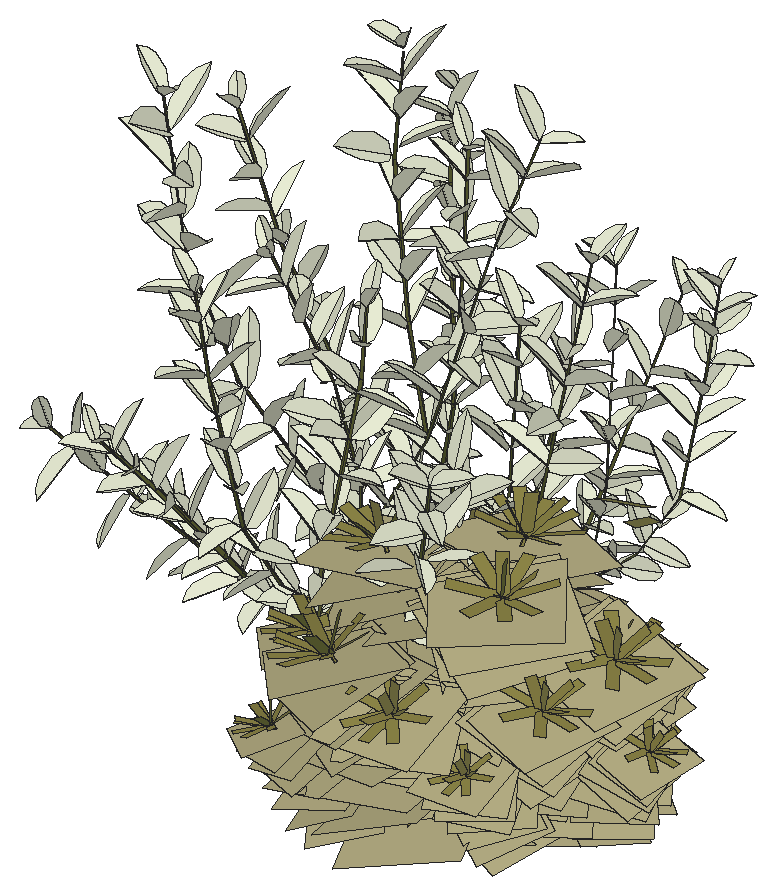
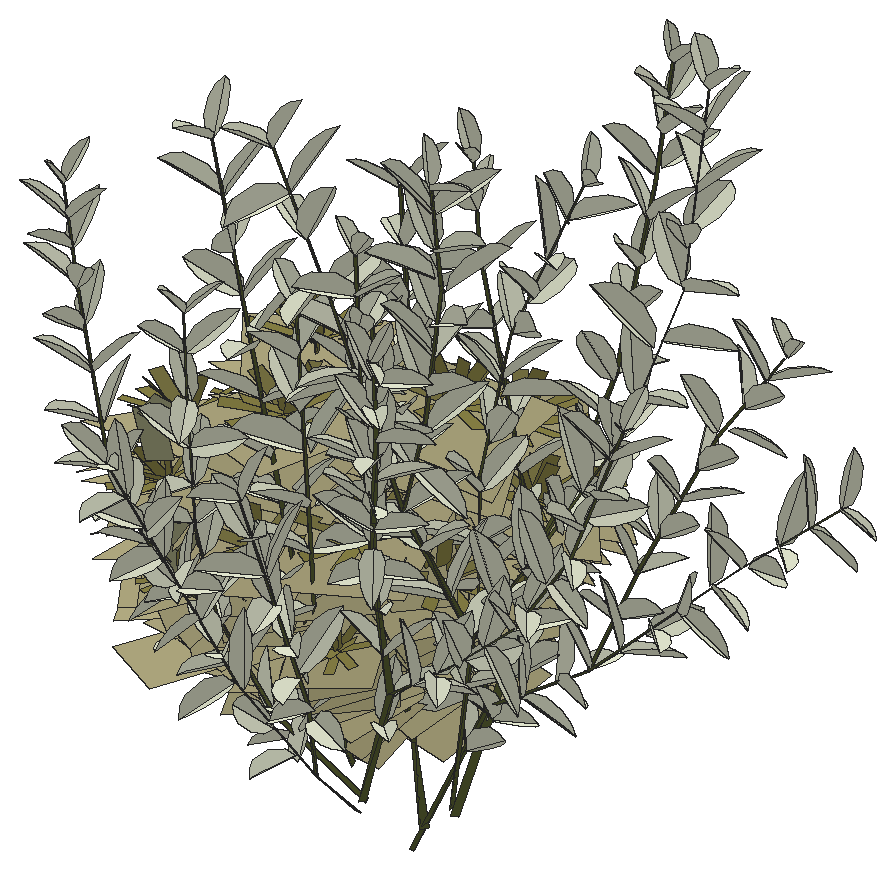
# SketchUp Ruby script. Lengths in inches.
U = 1.inch
M = Sketchup.active_model
def pt(a) = Geom::Point3d.new(a.map { |v| v * U })
def face(e, loops, mat)
  f = e.add_face(loops[0].map { |a| pt(a) })
  loops[1..].each { |l| e.add_face(l.map { |a| pt(a) }).erase! }
  f.material = f.back_material = mat if mat
  f
end
# faces: each face lists its corners as indices into pts; further lists are holes
def faces(e, pts, list, mat = nil) = list.each { |f| face(e, (f[0].is_a?(Array) ? f : [f]).map { |l| l.map { |i| pts[i] } }, mat) }
# xy, xz, yz: faces in a plane at the given z, y or x. An outline is a flat list of corners, or four numbers for a rectangle; further outlines are holes
def ring(l) = l.size == 4 ? [[l[0], l[1]], [l[2], l[1]], [l[2], l[3]], [l[0], l[3]]] : l.each_slice(2).to_a
def flat(e, list, mat, &to3) = list.each { |f| face(e, (f[0].is_a?(Array) ? f : [f]).map { |l| ring(l).map { |u, v| to3.(u, v) } }, mat) }
def xy(e, z, list, mat = nil) = flat(e, list, mat) { |x, y| [x, y, z] }
def xz(e, y, list, mat = nil) = flat(e, list, mat) { |x, z| [x, y, z] }
def yz(e, x, list, mat = nil) = flat(e, list, mat) { |y, z| [x, y, z] }
def lines(e, pts, list) = list.each { |a, b| e.add_line(pt(pts[a]), pt(pts[b])) }
# prism: a flat outline (further loops are holes) pulled along v
def prism(e, loops, v, mat = nil)
  f = face(e, loops, mat); d = Geom::Vector3d.new(v.map { |x| x * U })
  f.pushpull(f.normal.samedirection?(d) ? d.length : -d.length)
end
def box(e, o, s, mat = nil) = prism(e, [[o, [o[0] + s[0], o[1], o[2]], [o[0] + s[0], o[1] + s[1], o[2]], [o[0], o[1] + s[1], o[2]]]], [0, 0, s[2]], mat)
def at(x, y, z, deg = 0) = Geom::Transformation.translation(pt([x, y, z])) * Geom::Transformation.rotation(ORIGIN, Z_AXIS, deg.degrees)
def axes(o, x, y, z) = Geom::Transformation.new([*x, 0, *y, 0, *z, 0, *pt(o).to_a, 1])
def part(name) = M.definitions.add(name)
# library, detail: a bought-in or finely detailed component or shape, given as its bounding box
def library(name, o, s) = part(name).tap { |d| box(d.entities, o, s) }
def detail(e, o, s) = box(e.add_group.entities, o, s)
def put(e, d, t, mat = nil) = e.add_instance(d, t).tap { |i| i.material = mat if mat }
def group(e, t, mat = nil) = e.add_group.tap { |g| g.transformation = t; g.material = mat if mat }.entities
root = M.entities
M.materials.add("0ad16as01f6asdLeafVar1sfd015as60f1as6").color = [231, 235, 211]
M.materials.add("Colorsadfasdfa0sd1f06w3").color = [153, 130, 61]
M.materials.add("Euphorbia asdfasd0f150160s159w").color = [180, 173, 131]
M.materials.add("Euphorbiaasdfa0sdf1a56sd016wow Leaf SU").color = [141, 134, 72]
M.materials.add("asdfasdf0165f6asdLeafVar1sfd015as60f1as6").color = [231, 235, 211]
M.materials.add("dw_stemssadfasdfa0sdf1s01d6w1").color = [90, 97, 50]
M.materials.add("viburnumbladsadfasdfad0w122").color = [125, 129, 119]
c1 = part("vdw_leaf\#1")
p = [[0,0,0],[-2.77,1.61,2.32],[-4.3125,6.1,4.5],[-3.97,13.49,6.09],[-2.47,18.57,6.3],[-0.2,22.73,5.75],
  [2.54,19.66,6.85],[4.3,15.93,7.09],[5.03,7.6,5.43],[3.32,1.76,2.74]]
faces(c1.entities,p,[[0,1,2,3,4,5],[0,5,6,7,8,9]],"0ad16as01f6asdLeafVar1sfd015as60f1as6")
c2 = part("dw_branch_3\#2")
p = [[-10.06,-1.6,62.9],[-0.2,1.54,-0.01],[-10.43,1.54,62.72],[0.18,-1.6,0.17],[-23.75,-21.66,88.91],[-25.7,-20.3,89.55],
  [13.4,11.62,104.56],[13.33,13.52,104.47],[-49.25,-41.87,130.3125],[-50.33,-40.21,130.71],[-4.97,21.13,143.98],[35.61,27.99,178.64],
  [-5.09,23.64,143.96],[35.32,29.14,178.46],[-67.7,-55.38,181.06],[-68.34,-54.45,181.62],[-22.8125,33.9,200.59],[-22.94,35.79,200.41],
  [56.61,36.78,229.75],[56.29,38.09,229.57],[-70.63,-67.46,248.85],[-70.72,-66.33,249.5],[-25.05,43.32,240.75],[-24.98,44.26,240.57]]
faces(c2.entities,p,[[0,1,2],[0,3,1],[4,2,5],[4,0,2],[6,0,2],[6,2,7],[8,4,5],[8,5,9],
  [10,6,7],[11,6,7],[10,7,12],[11,7,13],[14,8,9],[14,9,15],[16,10,12],[16,12,17],
  [18,11,13],[18,13,19],[20,14,15],[20,15,21],[22,16,17],[22,17,23]],"dw_stemssadfasdfa0sdf1s01d6w1")
c3 = part("dw_branch3\#2")
put(c3.entities,c1,axes([-70.33,-63.58,233.32],[-1.00752,0.412,0.78596],[-0.24851,-1.22189,0.32195],[0.83141,0.09817,1.01433]))
put(c3.entities,c1,axes([-66.93,-54.91,182.82],[-0.84976,-0.98359,0.33619],[0.99572,-0.74889,0.32577],[-0.05223,0.46521,1.22907]))
put(c3.entities,c1,axes([-46.12,-39.49,126.35],[1.23843,0.5364,0.23552],[-0.56438,0.94474,0.81599],[0.15707,-0.83465,1.07498]))
put(c3.entities,c1,axes([13.0625,13.13,104.77],[-1.01271,0.69982,-0.26884],[-0.74268,-0.99813,0.19939],[-0.10222,0.31872,1.21473]))
put(c3.entities,c1,axes([-18.87,30.42,186.42],[0.36309,1.06515,-0.56675],[-1.14134,0.49515,0.19939],[0.39128,0.45593,1.10754]))
put(c3.entities,c1,axes([-3.2,4.15,75.77],[-1.04153,0.55414,0.44243],[-0.23365,-1.01045,0.71554],[0.6695,0.50943,0.93801]))
put(c3.entities,c1,axes([23.2,19.41,136.3],[-0.65687,-1.11295,-0.05714],[1.05857,-0.61429,-0.20411],[0.15163,-0.1536,1.24868]))
put(c3.entities,c1,axes([-25.57,35.48,201.32],[-0.64726,0.62827,0.87973],[-0.71635,-1.0172,0.19939],[0.80962,-0.39773,0.87973]))
put(c3.entities,c1,axes([-36.37,-32.14,110.35],[-0.80747,1.09962,0.12544],[-0.83333,-0.50188,-0.96467],[-0.72833,-0.64487,0.96467]))
put(c3.entities,c1,axes([-9.89,26.72,156.79],[0.45529,1.02969,0.56572],[-1.16919,0.33753,0.32662],[0.11537,-0.64297,1.07744]))
put(c3.entities,c1,axes([-26.57,46.1,241.0625],[0.00015,0.80921,0.22536],[-0.83985,0.00446,-0.01542],[-0.01605,-0.22532,0.80906]))
put(c3.entities,c1,axes([-9.2,-2.58,61.06],[-1.10001,-0.40312,0.39014],[0.40883,-1.1116,0.00411],[0.35732,0.13566,1.14763]))
put(c3.entities,c1,axes([-69.91,-63.11,233.93],[1.36249,-0.1432,0],[0.13201,1.25603,0.5309],[-0.05549,-0.52799,1.26295]))
put(c3.entities,c1,axes([32.2,25.46,166.13],[0.06878,-1.29051,-0.05714],[1.22165,0.07415,-0.20411],[0.2113,-0.04403,1.24868]))
put(c3.entities,c1,axes([-5.68,-0.66,44.43],[-0.48448,-1.12287,0.17078],[0.98138,-0.33653,0.57135],[-0.48308,0.36756,1.04626]))
put(c3.entities,c1,axes([43.45,32.81,198.64],[0.5408,1.19584,0.14106],[-0.94242,0.32409,0.86557],[0.74952,-0.45533,0.98656]))
put(c3.entities,c1,axes([12.52,14.14,104.98],[1.02694,0.54888,0.41092],[-0.53566,1.05407,-0.06927],[-0.38969,-0.12321,1.13846]))
put(c3.entities,c1,axes([44.55,32.375,198.73],[-0.65687,-1.11295,-0.05714],[1.05857,-0.61429,-0.20411],[0.15163,-0.1536,1.24868]))
put(c3.entities,c1,axes([-5.67,21.17,141.44],[-1.10726,0.43603,-0.32953],[-0.49537,-1.03435,0.29588],[-0.17521,0.40597,1.12589]))
put(c3.entities,c1,axes([55.69,37.84,229.48],[0.18984,0.96334,0.18958],[-0.71996,0.0053,0.69399],[0.66755,-0.26823,0.69457]))
put(c3.entities,c1,axes([-21.52,36.85,205.2],[0.72606,-0.98817,0.14519],[0.94364,0.7084,0.10251],[-0.16885,0.05176,1.19664]))
put(c3.entities,c1,axes([-68.51,-56.35,196.07],[1.16319,0.72381,0],[-0.66725,1.0723,0.5309],[0.28049,-0.45075,1.26295]))
put(c3.entities,c2,at(0.01,-0.09,-0.02),"dw_stemssadfasdfa0sdf1s01d6w1")
put(c3.entities,c1,axes([-2.49,5.18,75.91],[0.78614,-0.90346,-0.30078],[0.86953,0.79562,-0.11715],[0.28546,-0.14014,1.16705]))
put(c3.entities,c1,axes([-23.125,-16.22,82.25],[0.32175,1.32576,0.12544],[-1.33153,0.31835,0.05068],[0.01989,-0.13382,1.3633]))
put(c3.entities,c1,axes([-23.75,41.99,230.3],[0.85958,-0.87451,0.14519],[0.66531,0.75721,0.62192],[-0.54076,-0.36226,1.01955]))
put(c3.entities,c1,axes([27.07,22.48,149.34],[0.92952,-0.64745,-0.62467],[0.50188,1.074,-0.36637],[0.71693,0.02135,1.04468]))
put(c3.entities,c1,axes([17.66,16.25,119.93],[-0.91649,0.83891,-0.3601],[-0.87434,-0.77966,0.40896],[0.0492,0.54447,1.14321]))
put(c3.entities,c1,axes([-68.37,-54.54,181.63],[0.32047,1.28399,0.35434],[-1.33153,0.31835,0.05068],[-0.03484,-0.35624,1.32241]))
put(c3.entities,c1,axes([-28.98,-27.1,96.48],[-0.8814,-0.35966,-0.98523],[0.75246,-1.11336,-0.26672],[-0.73065,-0.71272,0.91382]))
put(c3.entities,c1,axes([-15.23,28.43,172.72],[-1.21149,0.11898,0.32517],[-0.09739,-1.25259,0.09551],[0.33228,0.0667,1.21356]))
put(c3.entities,c1,axes([-17.5625,31.23,186.85],[-0.49275,-1.12287,0.14519],[0.95014,-0.33653,0.62192],[-0.53717,0.36756,1.01955]))
put(c3.entities,c1,axes([26.7,21.22,149.39],[-1.00104,0.22334,0.83093],[0.36894,-1.0402,0.72406],[0.77731,0.78134,0.72643]))
put(c3.entities,c1,axes([-31.125,-24.87,97.38],[0.75482,-0.86936,0.69068],[-0.00159,0.80023,1.00899],[-1.08766,-0.58016,0.45842]))
put(c3.entities,c1,axes([-71.21,-66.73,248.67],[0.25207,0.96771,0],[-0.8921,0.23237,0.38752],[0.375,-0.09768,0.92186]))
put(c3.entities,c1,axes([-24.11,41.05,229.55],[-1.11612,0.51924,-0.26884],[-0.56394,-1.10897,0.19939],[-0.15444,0.29694,1.21473]))
put(c3.entities,c1,axes([6.75,8.37,91.63],[-0.33418,-1.12287,0.39014],[1.13558,-0.33653,0.00411],[0.10478,0.36756,1.14763]))
put(c3.entities,c1,axes([-26,45.89,241.63],[-0.26986,-0.70824,-0.32129],[0.56818,-0.39091,0.38449],[-0.49365,-0.09775,0.63011]))
put(c3.entities,c1,axes([3.74,17.32,124.35],[0.22441,1.22913,-0.16274],[-1.07812,0.11178,-0.64246],[-0.61228,0.25367,1.07162]))
put(c3.entities,c1,axes([-5.44,22.27,140.88],[1.2203,0.00475,0.31374],[-0.097,1.20386,0.35905],[-0.29841,-0.37189,1.1663]))
put(c3.entities,c1,axes([-13.79,29.35,173.31],[0.83169,-0.90108,0.14519],[0.68877,0.73594,0.62192],[-0.55187,-0.34509,1.01955]))
put(c3.entities,c1,axes([-16.92,-7.26,72.98],[1.30647,0.30378,-0.27886],[0.07026,0.74892,1.14503],[0.40633,-1.10623,0.69861]))
put(c3.entities,c1,axes([4.8,17.55,125.22],[-0.25598,-1.17842,0.26559],[1.01553,-0.08455,0.60363],[-0.56975,0.35087,1.00767]))
put(c3.entities,c1,axes([5.3125,8.35,91.45],[0.00638,1.22913,-0.27714],[-1.16413,0.11178,0.46895],[0.48205,0.25367,1.13617]))
put(c3.entities,c1,axes([38.12,30.57,183.07],[1.12534,0.26182,-0.63833],[-0.46674,1.18829,-0.33545],[0.5081,0.51169,1.10563]))
put(c3.entities,c1,axes([-70.41,-60.38,214.47],[-0.41425,1.30587,0],[-1.20383,-0.38188,0.5309],[0.50605,0.16053,1.26295]))
put(c3.entities,c1,axes([37.03,28.75,180.67],[-1.12533,0.00102,-0.63799],[-0.00113,-1.2408,0],[-0.62497,0.00057,1.10237]))
put(c3.entities,c1,axes([30.71,25.35,165.96],[-0.1364,1.29314,0.22715],[-1.08768,-0.23921,0.70862],[0.73536,-0.11394,1.09026]))
put(c3.entities,c1,axes([-38.05,-30.84,110.67],[-0.31533,-1.27379,-0.2839],[1.018,-0.40311,0.67794],[-0.74394,-0.05723,1.08307]))
put(c3.entities,c1,axes([50.11,34.45,213.36],[-1.05669,0.74401,-0.05714],[-0.616,-0.82138,0.69675],[0.37221,0.60904,1.04705]))
put(c3.entities,c1,axes([-65.32,-58.78,200.07],[-1.14597,-0.19668,-0.6713],[0.21784,-1.26924,0],[-0.64812,-0.11124,1.139]))
put(c3.entities,c1,axes([-53.2,-43.37,143.59],[-0.72817,-1.09167,-0.2839],[0.82127,-0.72411,0.67794],[-0.71934,0.19815,1.08307]))
put(c3.entities,c1,axes([-61.1,-50.25,163.67],[-0.52887,1.19686,-0.30066],[-1.10762,-0.57104,-0.32484],[-0.42634,0.12264,1.23812]))
put(c3.entities,c1,axes([-54.12,-42.96,142.67],[0.32175,1.32576,0.12544],[-1.33153,0.31835,0.05068],[0.01989,-0.13382,1.3633]))
put(c3.entities,c1,axes([22.03,20.08,132.3],[1.17066,0.5058,-0.34078],[-0.35758,1.16671,0.50333],[0.49407,-0.35407,1.17172]))
put(c3.entities,c1,axes([-8.59,26.04,158.21],[-0.49275,-1.12287,0.14519],[0.95014,-0.33653,0.62192],[-0.53717,0.36756,1.01955]))
put(c3.entities,c1,axes([49.92,34.03,213.7],[1.24742,-0.35176,0.25024],[0.42127,1.159,-0.4708],[-0.09426,0.52477,1.20753]))
put(c3.entities,c1,axes([-70.34,-67.02,249.05],[-0.57048,-0.79684,0],[0.73827,-0.52855,0.24329],[-0.20203,0.14464,0.92729]))
put(c3.entities,c1,axes([56.04,36.81,228.63],[0.33451,-0.90845,-0.15237],[0.87636,0.33365,-0.06538],[0.11487,-0.11636,0.94597]))
put(c3.entities,c1,axes([-69.93,-60.58,214.88],[-0.45293,-0.99272,-0.78227],[1.14635,-0.58199,0.07483],[-0.40282,-0.65636,1.06615]))
put(c3.entities,c1,axes([-16.77,-8.59,72.7],[-1.22785,0.11509,0.53076],[-0.24879,-1.22495,-0.30991],[0.46742,-0.38989,1.16587]))
put(c3.entities,c1,axes([18.29,17.18,119.24],[1.19981,-0.45946,0.3029],[0.40159,1.22775,0.27158],[-0.37626,-0.1547,1.25575]))
put(c3.entities,c1,axes([-6.73,-0.68,43.74],[0.05346,1.22913,-0.27201],[-1.22696,0.11178,0.26396],[0.28163,0.25367,1.20164]))
put(c3.entities,c1,axes([-58.57,-48.42,160.98],[0.43385,-1.23789,0.39533],[1.04879,0.57965,0.66404],[-0.76727,0.09236,1.13122]))
put(c3.entities,c1,axes([-23.4,38.49,215.38],[0.06762,1.22913,-0.26884],[-1.23909,0.11178,0.19939],[0.21835,0.25367,1.21473]))
put(c3.entities,c1,axes([-22.21,-16.62,83.17],[-0.72817,-1.09167,-0.2839],[0.82127,-0.72411,0.67794],[-0.71934,0.19815,1.08307]))
put(c3.entities,c1,axes([-45.7,-40.77,126.53],[-1.33715,-0.0713,-0.0976],[0.07167,-1.28508,-0.04314],[-0.09306,-0.0492,1.31098]))
put(c3.entities,c1,axes([-22.39,38.51,216.12],[-0.49275,-1.12287,0.14519],[0.95014,-0.33653,0.62192],[-0.53717,0.36756,1.01955]))
c4 = part("vdw_leaf\#2")
p = [[0,0,0],[-2.77,1.61,2.32],[-4.3125,6.1,4.5],[-3.97,13.49,6.09],[-2.47,18.57,6.3],[-0.2,22.73,5.75],
  [2.54,19.66,6.85],[4.3,15.93,7.09],[5.03,7.6,5.43],[3.32,1.76,2.74]]
faces(c4.entities,p,[[0,1,2,3,4,5],[0,5,6,7,8,9]],"asdfasdf0165f6asdLeafVar1sfd015as60f1as6")
c5 = part("dg_branch_1\#2")
p = [[46.12,1.57,35.62],[46,5.42,35.41],[0.14,1.79,0.05],[0.26,-2.0625,0.27],[74.05,2.99,75.8],[74.11,5.28,75.58],
  [103.46,0.47,94.74],[104.03,2.92,94.84],[81.14,16.92,120.46],[81.2,18.78,120.24],[130.47,-5.6875,130.27],[130.58,-3.66,129.85],
  [80.82,34.4375,191.22],[80.64,35.93,190.9],[148.49,-14.56,203.24],[148.9,-12.8125,203.11],[81.08,37.95,226.93],[81.4,39.1,227.03],
  [157.45,-18.19,250.77],[157.7,-17.01,250.41]]
faces(c5.entities,p,[[0,1,2,3],[4,0,1],[4,1,5],[6,4,5],[6,5,7],[8,4,5],[8,5,9],[10,6,7],
  [10,7,11],[12,8,9],[12,9,13],[14,10,11],[14,11,15],[16,12,13],[16,13,17],[18,14,15],
  [18,15,19]],"dw_stemssadfasdfa0sdf1s01d6w1")
c6 = part("vdw_branch1\#3")
put(c6.entities,c4,axes([120.69,-2.42,117.31],[1.12221,-0.24063,-0.65809],[0.19207,1.24776,-0.12871],[0.65778,0.01392,1.11658]))
put(c6.entities,c4,axes([81,38.9,226.05],[0.7888,-0.58155,0],[0.48308,0.65523,0.47],[-0.28484,-0.38635,0.83138]))
put(c6.entities,c4,axes([78.08,12.69,106.05],[-1.43826,-0.02353,-0.03177],[0.0088,-1.31777,0.57755],[-0.03854,0.57714,1.31741]))
put(c6.entities,c4,axes([130.18,-4.73,130.41],[-0.38031,-1.29044,-0.11242],[1.20662,-0.31032,-0.51987],[0.47109,-0.24694,1.24081]))
put(c6.entities,c4,axes([157.08,-17.89,249.93],[-0.91355,0.40674,0],[-0.37496,-0.84216,0.38752],[0.15762,0.35401,0.92186]))
put(c6.entities,c4,axes([90.64,3.03,86.49],[0.32514,-0.85045,-0.99675],[0.69523,0.98247,-0.61148],[1.11061,-0.36604,0.67459]))
put(c6.entities,c4,axes([80.15,28.42,160.95],[-0.16039,0.95636,-1.06292],[-1.41646,0.03966,0.24943],[0.19509,1.07422,0.93709]))
put(c6.entities,c4,axes([126.74,-5.45,129.22],[-0.59819,0.96152,-0.6841],[-0.85772,0.12575,0.92675],[0.75427,0.88089,0.57856]))
put(c6.entities,c4,axes([133.22,-6.12,150.66],[-0.93823,0.76985,0.59124],[-0.47726,-1.08188,0.65135],[0.84525,0.24366,1.02405]))
put(c6.entities,c4,axes([80.43,22.89,141.32],[-1.42571,-0.19312,0.01373],[0.18338,-1.31425,0.5561],[-0.0621,0.5528,1.32692]))
put(c6.entities,c4,axes([33.14,0.88,26.42],[-0.13338,1.31536,0.04876],[-1.04528,-0.13221,0.7073],[0.72315,0.03348,1.07497]))
put(c6.entities,c4,axes([152.63,-15.08,221.76],[-1.28188,0.41945,0.0579],[-0.3638,-1.18547,0.53367],[0.21665,0.49113,1.23869]))
put(c6.entities,c4,axes([80.05,28.28,160.33],[-0.46732,-1.26661,0.40679],[1.27397,-0.40257,0.21004],[-0.07408,0.44645,1.30501]))
put(c6.entities,c4,axes([153.95,-14.8,235.875],[0.39005,1.07743,0.20605],[-0.96443,0.25296,0.50293],[0.42961,-0.3464,0.99807]))
put(c6.entities,c4,axes([80.2,24.22,141.74],[1.33062,-0.46576,0.02628],[0.44746,1.2746,-0.06608],[-0.00197,0.0722,1.37936]))
put(c6.entities,c4,axes([145.48,-12.5,188.92],[-1.32952,0.16983,0.16138],[-0.09299,-1.2361,0.53471],[0.21503,0.51548,1.22904]))
put(c6.entities,c4,axes([139.64,-9.18,171.24],[0.05682,1.30088,0.23414],[-1.13176,-0.05343,0.57151],[0.58357,-0.22963,1.13417]))
put(c6.entities,c4,axes([70.95,4.35,71.98],[-1.1081,-0.41873,0.64752],[0.33675,-1.28259,-0.25313],[0.6937,-0.04625,1.15721]))
put(c6.entities,c4,axes([59.85,4.55,56.17],[-0.26797,1.24526,0.35754],[-0.9369,-0.41634,0.74783],[0.83377,-0.10389,0.98674]))
put(c6.entities,c4,axes([33.11,3.36,25.66],[-0.57817,-1.07968,-0.5679],[1.11554,-0.21356,-0.7297],[0.49375,-0.78178,0.98363]))
put(c6.entities,c5,at(-0.21,0.34,-0.17),"dw_stemssadfasdfa0sdf1s01d6w1")
put(c6.entities,c4,axes([80.91,19.01,122.53],[-0.84258,1.13222,-0.27981],[-1.15093,-0.75138,0.42537],[0.18861,0.47293,1.3457]))
put(c6.entities,c4,axes([119.8,-1.22,114.1],[-1.3235,-0.25012,0.09101],[0.25933,-1.31572,0.15537],[0.05991,0.1698,1.33794]))
put(c6.entities,c4,axes([46.29,5.1,38.04],[0.98937,0.73827,-0.47585],[-0.72359,1.03721,0.10473],[0.44068,0.18581,1.20453]))
put(c6.entities,c4,axes([81.1875,33.03,184.45],[1.33883,0.26986,0.35053],[-0.09581,1.22087,-0.57399],[-0.42216,0.53228,1.20262]))
put(c6.entities,c4,axes([80.16,36.28,206.98],[-0.83993,0.85737,-0.6234],[-1.05964,-0.65701,0.5241],[0.02941,0.81391,1.07976]))
put(c6.entities,c4,axes([154.86,-16.15,234.87],[0.02509,-1.15302,-0.28506],[1.1487,-0.04894,0.29908],[-0.30202,-0.28195,1.11384]))
put(c6.entities,c4,axes([108.77,-0.33,101.14],[-0.47691,-1.03266,-0.72709],[1.25395,-0.29455,-0.40416],[0.15052,-0.81814,1.06325]))
put(c6.entities,c4,axes([89.79,3.01,85.87],[-0.61344,0.75518,0.8965],[-0.17758,-1.01824,0.73622],[1.13385,0.22574,0.58569]))
put(c6.entities,c4,axes([81.56,20.31,123.29],[0.37259,-1.3435,0.21057],[1.29385,0.32364,-0.22445],[0.16906,0.25791,1.34638]))
put(c6.entities,c4,axes([46.45,1.82,36.74],[-0.77883,0.29892,1.0614],[0.19124,-1.24314,0.49044],[1.08598,0.43329,0.67484]))
put(c6.entities,c4,axes([71.37,4.02,72.32],[0.72905,0.81546,-0.74421],[-0.66805,0.98958,0.42988],[0.8391,0.14186,0.97745]))
put(c6.entities,c4,axes([136.59,-5.88,150.53],[0.85845,-0.99897,-0.12437],[0.96526,0.81273,0.13453],[-0.02572,-0.18182,1.28292]))
put(c6.entities,c4,axes([80.375,38.8,225.86],[-0.25178,0.96778,0],[-0.89216,-0.23211,0.38752],[0.37503,0.09757,0.92186]))
put(c6.entities,c4,axes([74.43,7.99,85.38],[-1.05703,0.91669,-0.33543],[-0.95806,-0.87958,0.61531],[0.18697,0.6754,1.25659]))
put(c6.entities,c4,axes([76.57,9.74,89.32],[0.63146,-1.21538,0.33508],[1.18148,0.49387,-0.43517],[0.26321,0.48577,1.26593]))
put(c6.entities,c4,axes([81.6875,36.97,207.4],[0.09422,-1.04424,0.38486],[1.01646,0.1939,0.27727],[-0.33299,0.33382,0.98727]))
put(c6.entities,c4,axes([157.29,-17.17,249.98],[0.50586,-0.50586,0],[0.38853,0.38853,0.41105],[-0.29684,-0.29684,0.56115]))
put(c6.entities,c4,axes([79.92,15.8,106.09],[1.03917,-0.29343,-0.90675],[-0.14587,1.22131,-0.5624],[0.92163,0.5191,0.88824]))
put(c6.entities,c4,axes([61.95,3.88,56.26],[0.41243,-1.28546,0],[1.17466,0.37688,-0.54831],[0.5221,0.16751,1.23363]))
put(c6.entities,c4,axes([151.99,-14.79,208.15],[-0.48571,-1.21723,-0.32393],[1.25386,-0.50033,0],[-0.12005,-0.30087,1.31056]))
put(c6.entities,c4,axes([108.44,0.62,102.22],[0.82183,0.96078,0.38967],[-0.62327,0.08618,1.10203],[0.79141,-0.88661,0.51693]))
put(c6.entities,c4,axes([145.6,-10.56,188.62],[1.03241,-0.02554,-0.82693],[0.3944,1.11584,0.45794],[0.70325,-0.61672,0.89706]))
put(c6.entities,c4,axes([78.59,32.3,183.89],[-1.12675,-0.42036,0.43987],[0.5899,-0.98149,0.57312],[0.14901,0.70693,1.05726]))
put(c6.entities,c4,axes([152.08,-13.42,223.37],[0.79993,-0.44251,-0.69938],[0.68456,0.82615,0.26026],[0.41048,-0.60953,0.85515]))
put(c6.entities,c4,axes([140.71,-8.74,170.55],[0.41903,-1.24177,-0.32393],[1.26224,0.33728,0.33986],[-0.23168,-0.40836,1.26573]))
put(c6.entities,c4,axes([149.25,-12.53,205.78],[1.24456,0.38285,0.23414],[-0.42999,1.04826,0.57151],[-0.02056,-0.62679,1.13417]))
c7 = part("vdw_leaf\#3")
p = [[0,0,0],[-2.77,1.61,2.32],[-4.3125,6.1,4.5],[-3.97,13.49,6.09],[-2.47,18.57,6.3],[-0.2,22.73,5.75],
  [2.54,19.66,6.85],[4.3,15.93,7.09],[5.03,7.6,5.43],[3.32,1.76,2.74]]
faces(c7.entities,p,[[0,1,2,3,4,5],[0,5,6,7,8,9]],"asdfasdf0165f6asdLeafVar1sfd015as60f1as6")
c8 = part("dw_brancj_2\#2")
p = [[9.7,-0.22,29.95],[0.23,-1.96,0.34],[-0.05,1.51,0.11],[9.65,1.51,29.46],[18.64,-8.75,84.43],[18.96,-6.63,84.625],
  [1.53,6.02,63.68],[1.42,8.18,63.25],[-10.58,8.77,161.17],[-10.41,9.98,160.68],[26.34,-9.37,211.72],[26.57,-8.28,211.23]]
faces(c8.entities,p,[[0,1,2],[0,2,3],[4,0,3],[4,3,5],[6,0,3],[6,3,7],[8,6,7],[8,7,9],
  [10,4,5],[10,5,11]],"dw_stemssadfasdfa0sdf1s01d6w1")
c9 = part("vdw_branch2\#3")
put(c9.entities,c7,axes([19.53,-5.9,102.42],[1.12377,-0.50004,0],[0.46097,1.03596,0.47664],[-0.19377,-0.43548,1.13389]))
put(c9.entities,c7,axes([-5.89,6.52,109.44],[-1.07209,0.83679,0],[-0.77141,-0.98832,0.52702],[0.32427,0.41545,1.25373]))
put(c9.entities,c7,axes([-0.44,8.23,75.28],[0.88709,-0.9947,0],[0.92159,0.82189,0.33087],[-0.25219,-0.22491,1.26111]))
put(c9.entities,c7,axes([24.71,-8.97,190.81],[-0.82641,0.91101,0],[-0.83983,-0.76184,0.47664],[0.35303,0.32025,1.13389]))
put(c9.entities,c7,axes([-2.29,8.24,91.35],[1.24603,-0.47303,0],[0.43826,1.15445,0.33087],[-0.11993,-0.31592,1.26111]))
put(c9.entities,c7,axes([12.26,-3.11,37.92],[-0.64625,1.02205,0.22511],[-1.04383,-0.61044,-0.22511],[-0.07533,-0.30931,1.18809]))
put(c9.entities,c7,axes([26.17,-9.17,210.27],[-0.99452,-0.10453,0],[0.09636,-0.91681,0.38752],[-0.04051,0.38539,0.92186]))
put(c9.entities,c7,axes([-6.07,9.4,125.35],[-0.90214,-0.98107,0],[0.90896,-0.83583,0.33087],[-0.24874,0.22873,1.26111]))
put(c9.entities,c7,axes([-4.13,7.29,110.58],[0.44715,-1.078,0.64369],[1.05816,0.63649,0.33087],[-0.58725,0.40856,1.09216]))
put(c9.entities,c7,axes([23.91,-8.22,171.96],[0.62307,0.85009,-0.63406],[-0.71531,0.8798,0.47664],[0.78296,0.12729,0.94004]))
put(c9.entities,c8,at(-0.09,0.18,-0.25),"dw_stemssadfasdfa0sdf1s01d6w1")
put(c9.entities,c7,axes([23.34,-9.65,156.59],[-0.31364,-1.00782,0.58216],[1.10369,-0.17062,0.29925],[-0.17137,0.6239,0.98776]))
put(c9.entities,c7,axes([15.03,-3.37,58.83],[-1.05425,-0.00194,0.58442],[-0.14303,-1.11707,-0.26172],[0.55355,-0.3046,0.99755]))
put(c9.entities,c7,axes([-11.625,9.46,160.37],[0.36812,0.92978,0],[-0.85713,0.33936,0.38752],[0.3603,-0.14265,0.92186]))
put(c9.entities,c7,axes([21.32,-8.53,138.72],[1.21379,0.19904,0],[-0.19904,1.21379,0],[0,0,1.23]))
put(c9.entities,c7,axes([22.54,-9.2,141.43],[-1.02887,0.17955,0.60182],[-0.23387,-1.13057,-0.06253],[0.56696,-0.17376,1.02111]))
put(c9.entities,c7,axes([23.9,-8.82,173.84],[-1.14567,-0.37474,0],[0.35918,-1.0981,0.04438],[-0.01409,0.04308,1.17993]))
put(c9.entities,c7,axes([-7.84,8.92,143.59],[-1.26971,0.40522,0],[-0.37543,-1.17638,0.33087],[0.10274,0.32192,1.26111]))
put(c9.entities,c7,axes([19.77,-8.01,85.98],[-0.32405,-1.14591,0.18674],[1.10278,-0.32969,-0.10948],[0.15845,0.14442,1.16117]))
put(c9.entities,c7,axes([-0.62,5.76,76.34],[-0.08879,1.17576,-0.67771],[-1.34525,-0.16582,-0.11144],[-0.17897,0.66309,1.17383]))
put(c9.entities,c7,axes([20.49,-8.22,121.07],[0.39924,-0.78471,-0.8233],[1.08735,0.33121,0.2116],[0.09035,-0.83005,0.83495]))
put(c9.entities,c7,axes([15.15,-3.72,62.9],[1.16251,0.40128,-0.0211],[-0.39924,1.16074,0.07874],[0.0456,-0.06757,1.2273]))
put(c9.entities,c7,axes([20.72,-8.08,120.26],[-0.03693,1.2277,-0.06551],[-1.22944,-0.03698,0],[-0.00197,0.06548,1.22825]))
put(c9.entities,c7,axes([22.58,-8.36,155.57],[-0.56247,1.09386,0],[-1.00839,-0.51852,0.47664],[0.42389,0.21796,1.13389]))
put(c9.entities,c7,axes([3.97,3.13,57.96],[-1.09459,0.76041,0],[-0.72262,-1.0402,-0.1735],[-0.10109,-0.14552,1.29352]))
put(c9.entities,c7,axes([-10.8,9.06,160.75],[-0.66334,-0.72138,0],[0.66835,-0.61458,0.24329],[-0.1829,0.16818,0.92729]))
put(c9.entities,c7,axes([19.06,-9.3125,103.96],[-1.01345,0.25553,-0.60051],[-0.2265,-1.12952,-0.09839],[-0.59598,0.03076,1.01889]))
put(c9.entities,c7,axes([18.07,-6.2,81.7],[-0.56247,1.09386,0],[-1.00839,-0.51852,0.47664],[0.42389,0.21796,1.13389]))
put(c9.entities,c7,axes([12.95,-0.39,43.31],[0.13044,-1.19832,0],[1.11025,0.12085,0.29925],[-0.30382,-0.03307,1.14057]))
put(c9.entities,c7,axes([2.28,8.28,56.18],[1.32413,-0.31027,0],[0.30923,1.31968,-0.11144],[0.02542,0.1085,1.35543]))
put(c9.entities,c7,axes([-7.55,9.96,143.07],[1.34251,-0.21744,0],[0.20045,1.23761,0.52702],[-0.08426,-0.52024,1.25373]))
put(c9.entities,c7,axes([26.15,-8.25,210.66],[0.94661,-0.25364,0],[0.235,0.87703,0.24329],[-0.06431,-0.24,0.92729]))
put(c9.entities,c7,axes([-6.48,11.37,125.16],[0.64635,1.10315,0.46356],[-1.16569,0.46153,0.52702],[0.27017,-0.6478,1.16488]))
put(c9.entities,c7,axes([25.74,-8.35,191.28],[0.13044,-1.19832,0],[1.11025,0.12085,0.29925],[-0.30382,-0.03307,1.14057]))
put(c9.entities,c7,axes([-5.125,7.47,91.6],[-1.10024,0.63688,0.48318],[-0.78682,-1.00808,-0.46292],[0.14137,-0.65404,1.184]))
c10 = part("Component\#306")
p = [[4.55,0.11,0],[4.55,0,0],[2.84,0,3.13],[2.84,0.11,3.13],[4.625,0.05,0.04],[2.92,0.05,3.15],
  [2.08,0,8.07],[2.08,0.11,8.07],[2.16,0.05,8.1],[0,0,12.54],[0,0.11,12.54],[0.07,0.05,12.58]]
faces(c10.entities,p,[[0,1,2,3],[1,4,5,2],[1,0,4],[4,0,3,5],[3,2,6,7],[2,5,8,6],[5,3,7,8],[7,6,9,10],
  [6,8,11,9],[8,7,10,11],[10,9,11]],"Colorsadfasdfa0sd1f06w3")
c11 = part("Component\#301")
xy(c11.entities,0,[[0,0,0.7,3.1]],"Euphorbiaasdfa0sdf1a56sd016wow Leaf SU")
c12 = part("Leaf rosette")
put(c12.entities,c11,axes([2.21,1.74,0.13],[-0.4441,0.47879,-0.0956],[-0.4878,-0.4406,0.05935],[-0.03146,0.16757,0.98536]))
put(c12.entities,c11,axes([2.29,1.9,0.17],[-0.62678,-0.10063,-0.18061],[0.01105,-0.59203,0.2915],[-0.31282,0.41486,0.85442]))
put(c12.entities,c11,axes([2.09,1.69,0.1],[-0.10438,0.65169,0],[-0.65169,-0.10438,0],[0,0,1]))
put(c12.entities,c11,axes([1.97,1.77,0.02],[0.31114,0.5228,0.25587],[-0.57125,0.32993,0.02052],[-0.16918,-0.3502,0.92127]))
put(c12.entities,c11,axes([1.93,1.95,0],[0.54816,-0.03215,0.36617],[-0.11878,0.60671,0.23108],[-0.52706,-0.39065,0.75472]))
put(c12.entities,c11,axes([2.04,2.1,0.05],[0.26275,-0.55867,0.23335],[0.34186,0.34684,0.44545],[-0.75711,-0.08556,0.64766]))
put(c12.entities,c11,axes([2.22,2.08,0.13],[-0.29265,-0.59104,-0.02512],[0.40323,-0.2198,0.47401],[-0.65583,0.2952,0.69479]))
c13 = part("Component\#308")
xy(c13.entities,0,[[0,0,5.01,4.64]],"Euphorbia asdfasd0f150160s159w")
c14 = part("Component\#316")
put(c14.entities,c10,at(2.35,3.5,0))
put(c14.entities,c12,at(0.25,1.59,12.45))
put(c14.entities,c13,axes([7.46,0.77,3.64],[0.10848,0.99337,0.03799],[-0.82378,0.11122,-0.55589],[-0.55643,0.02901,0.83038]))
put(c14.entities,c13,axes([1.97,2.58,1.93],[0.80762,-0.50565,0.30344],[0.47433,0.86274,0.17519],[-0.35038,0.00244,0.93661]))
put(c14.entities,c13,axes([5.79,0.14,3.9],[0.5013,0.78918,0.35482],[-0.74775,0.60146,-0.2813],[-0.4354,-0.1243,0.89162]))
put(c14.entities,c13,axes([1.87,2.6,3.75],[0.73154,-0.49698,0.46676],[0.47433,0.86274,0.17519],[-0.48976,0.09324,0.86686]))
put(c14.entities,c13,axes([3.91,7.06,6.66],[-0.50827,-0.83837,-0.19699],[0.8278,-0.53869,0.15675],[-0.23753,-0.08339,0.96779]))
put(c14.entities,c13,axes([1.2,3.99,6.83],[0.56066,-0.79708,0.22433],[0.74237,0.60386,0.29025],[-0.36682,0.0038,0.93028]))
put(c14.entities,c11,axes([2.42,3.73,12.57],[-0.1322,-0.64472,0.04955],[0.10064,0.02944,0.65162],[-0.9678,0.2092,0.14002]))
put(c14.entities,c11,axes([2.57,3.43,12.63],[-0.62833,0.089,-0.18134],[-0.19954,-0.36568,0.51192],[-0.04764,0.82148,0.56824]))
put(c14.entities,c13,axes([4.04,6.92,11.09],[-0.67411,-0.5063,-0.5378],[0.44628,-0.85937,0.24964],[-0.58857,-0.07172,0.80526]))
put(c14.entities,c11,axes([2.5,3.49,12.74],[-0.62833,0.089,-0.18134],[-0.18746,-0.03618,0.63178],[0.11402,0.98935,0.09049]))
put(c14.entities,c11,axes([2.3,3.27,12.51],[0.02916,0.64747,0.12464],[-0.56235,-0.04072,0.34308],[0.5216,-0.18387,0.83314]))
put(c14.entities,c13,axes([0.26,4.96,9.69],[0.33661,-0.92735,0.16343],[0.73504,0.36725,0.56995],[-0.58857,-0.07172,0.80526]))
put(c14.entities,c13,axes([4.76,6.31,12.62],[-0.95056,-0.1129,-0.28929],[0.09021,-0.99179,0.09066],[-0.29715,0.06008,0.95294]))
put(c14.entities,c13,axes([5.2,6.55,10.37],[-0.76372,-0.27738,-0.58291],[0.26517,-0.95808,0.10848],[-0.58857,-0.07172,0.80526]))
c15 = part("Plant stem")
p = [[2.84,0.11,3.13],[2.84,0,3.13],[2.08,0,8.07],[2.08,0.11,8.07],[2.92,0.05,3.15],[2.16,0.05,8.1],
  [0,0,12.54],[0,0.11,12.54],[0.07,0.05,12.58]]
faces(c15.entities,p,[[0,1,2,3],[1,4,5,2],[4,0,3,5],[3,2,6,7],[2,5,8,6],[5,3,7,8],[7,6,8]],"Colorsadfasdfa0sd1f06w3")
c16 = part("Leafy shoot")
put(c16.entities,c15,at(2.35,3.5,0))
put(c16.entities,c12,at(0.25,1.59,12.45))
put(c16.entities,c13,axes([1.87,2.6,3.75],[0.73154,-0.49698,0.46676],[0.47433,0.86274,0.17519],[-0.48976,0.09324,0.86686]))
put(c16.entities,c13,axes([3.91,7.06,6.66],[-0.50827,-0.83837,-0.19699],[0.8278,-0.53869,0.15675],[-0.23753,-0.08339,0.96779]))
put(c16.entities,c13,axes([1.2,3.99,6.83],[0.56066,-0.79708,0.22433],[0.74237,0.60386,0.29025],[-0.36682,0.0038,0.93028]))
put(c16.entities,c11,axes([2.42,3.73,12.57],[-0.1322,-0.64472,0.04955],[0.10064,0.02944,0.65162],[-0.9678,0.2092,0.14002]))
put(c16.entities,c11,axes([2.57,3.43,12.63],[-0.62833,0.089,-0.18134],[-0.19954,-0.36568,0.51192],[-0.04764,0.82148,0.56824]))
put(c16.entities,c13,axes([4.04,6.92,11.09],[-0.67411,-0.5063,-0.5378],[0.44628,-0.85937,0.24964],[-0.58857,-0.07172,0.80526]))
put(c16.entities,c11,axes([2.5,3.49,12.74],[-0.62833,0.089,-0.18134],[-0.18746,-0.03618,0.63178],[0.11402,0.98935,0.09049]))
put(c16.entities,c11,axes([2.3,3.27,12.51],[0.02916,0.64747,0.12464],[-0.56235,-0.04072,0.34308],[0.5216,-0.18387,0.83314]))
put(c16.entities,c13,axes([0.26,4.96,9.69],[0.33661,-0.92735,0.16343],[0.73504,0.36725,0.56995],[-0.58857,-0.07172,0.80526]))
put(c16.entities,c13,axes([4.76,6.31,12.62],[-0.95056,-0.1129,-0.28929],[0.09021,-0.99179,0.09066],[-0.29715,0.06008,0.95294]))
put(c16.entities,c13,axes([5.2,6.55,10.37],[-0.76372,-0.27738,-0.58291],[0.26517,-0.95808,0.10848],[-0.58857,-0.07172,0.80526]))
put(c16.entities,c13,axes([7.03,0.77,3.77],[0.19714,0.84663,0.32426],[-0.94994,0.28899,-0.30484],[-0.2731,-0.45173,0.91532]))
c17 = part("Groundcover plant")
put(c17.entities,c14,axes([0.82,1.83,0.8125],[0.98541,0,-0.17021],[0,1,0],[0.17021,0,0.98541]))
put(c17.entities,c16,axes([4.45,-0.84,-2.24],[0.69527,0.50616,0],[-0.50264,0.69042,-0.10135],[-0.05965,0.08194,0.85401]))
put(c17.entities,c16,axes([1.85,7.37,-3.38],[0.7038,-0.47341,0.14191],[0.46407,0.71797,0.09357],[-0.16999,0,0.84303]))
put(c17.entities,c16,axes([6.9,-3.65,-2.52],[0.79351,0.57769,0],[-0.57366,0.78798,-0.11567],[-0.06808,0.09351,0.97468]))
put(c17.entities,c16,axes([1.36,5.18,-2.66],[0.50674,-0.34086,0.10218],[0.33413,0.51694,0.06737],[-0.12239,0,0.60698]))
put(c17.entities,c16,axes([5.76,-1.49,-2.17],[0.43479,0.43181,0.07251],[-0.43488,0.43544,-0.06951],[-0.06212,-0.06169,0.61918]))
c18 = part("Groundcover clump")
put(c18.entities,c17,axes([25.06,6.72,0.82],[-0.74291,1.22188,0],[-1.22188,-0.74291,0],[0,0,1]))
put(c18.entities,c17,axes([-0.76,2.1875,0.82],[1.43,0,0],[0,1.43,0],[0,0,1]))
put(c18.entities,c17,axes([8.21,24.79,0.82],[-0.6403,-1.27864,0],[1.27864,-0.6403,0],[0,0,1]))
c19 = part("Component\#315")
p = [[0.25,0,0],[2.05,0.01,0.35],[1.81,4.2,1.66],[0,4.19,1.3125]]
faces(c19.entities,p,[[0,1,2,3]],"viburnumbladsadfasdfad0w122")
c20 = part("viburnumblad2")
put(c20.entities,c19,axes([-19.23,-4.49,-32.18],[83.35428,0,0],[0,79.38502,0],[0,0,83.35428]))
put(root,c3,axes([2170.53,276.4,10.58],[0.09481,-0.08589,0.04174],[0.08433,0.10034,0.02262],[-0.03765,0.00844,0.15579]))
put(root,c3,axes([2171.73,269.98,3.93],[-0.12304,0.0546,-0.04713],[-0.02701,-0.11428,-0.0937],[-0.06098,-0.05955,0.13659]))
put(root,c3,axes([2169.125,269.36,7.47],[0.1634,0,0],[0,0.1634,0],[0,0,0.20106]))
put(root,c6,axes([2168.67,269.59,7.1875],[0.01907,-0.13922,0],[0.13922,0.01907,0],[0,0,0.17291]))
put(root,c9,axes([2175.48,270.625,5.57],[0.02729,0.1244,-0.09048],[-0.14364,0.03151,0],[0.01575,0.07182,0.15671]))
put(root,c9,axes([2171.16,269.52,5.4],[0.09858,-0.0952,-0.10951],[0.11351,0.11754,0],[0.06402,-0.06182,0.16863]))
put(root,c9,axes([2176.39,269.95,8.3],[0.15791,0.02906,-0.03733],[-0.02958,0.1607,0],[0.02984,0.00549,0.19757]))
put(root,c6,axes([2174.15,271.36,7.18],[0.11749,0.04939,0],[-0.04939,0.11749,0],[0,0,0.15683]))
put(root,c18,axes([2167.64,243.65,7.84],[1.49047,0,0],[0,1.49047,0],[0,0,1.49047]))
put(root,c20,axes([2190.73,271.43,30.14],[0.00132,0.00974,-0.00592],[-0.01063,-0.00165,-0.00484],[-0.00451,0.00633,0.00719]))
put(root,c20,axes([2190.46,268.83,18.55],[0.00484,0.0109,0.00393],[-0.00707,0.00614,-0.00813],[-0.00911,0.00107,0.00791]))
put(root,c20,axes([2191.42,269.01,19.77],[-0.00591,0.00596,-0.00904],[-0.00601,-0.0106,-0.00307],[-0.00924,0.00313,0.00728]))
put(root,c20,axes([2190.88,270.73,28.82],[0.008,0.00859,-0.00017],[-0.00687,0.00594,-0.00742],[-0.00498,0.00541,0.0075]))
